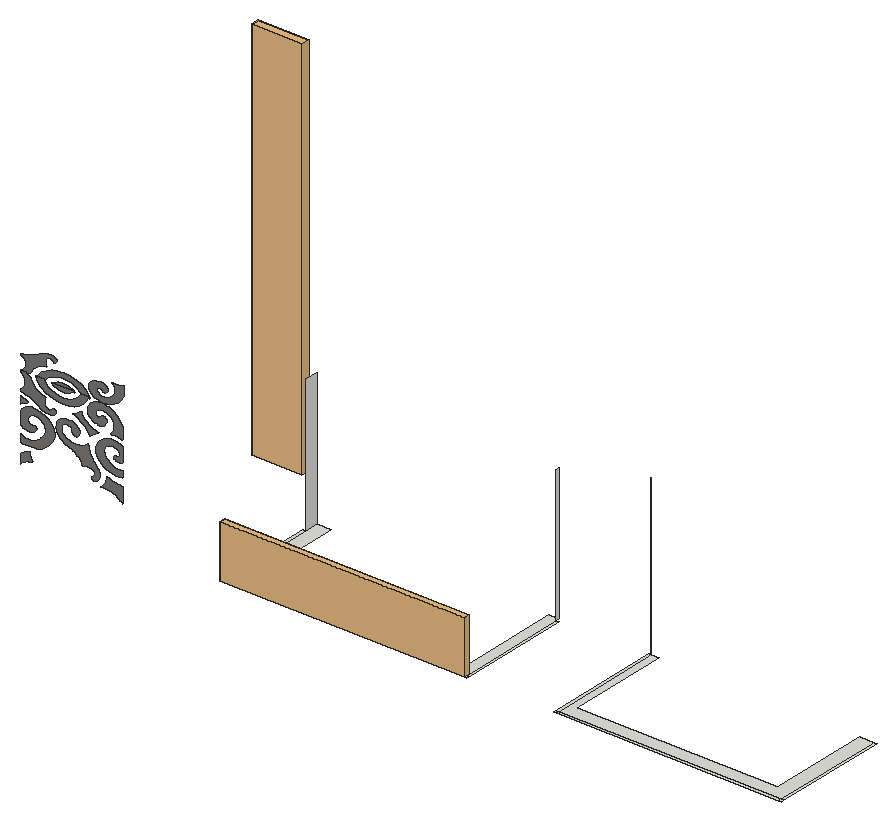
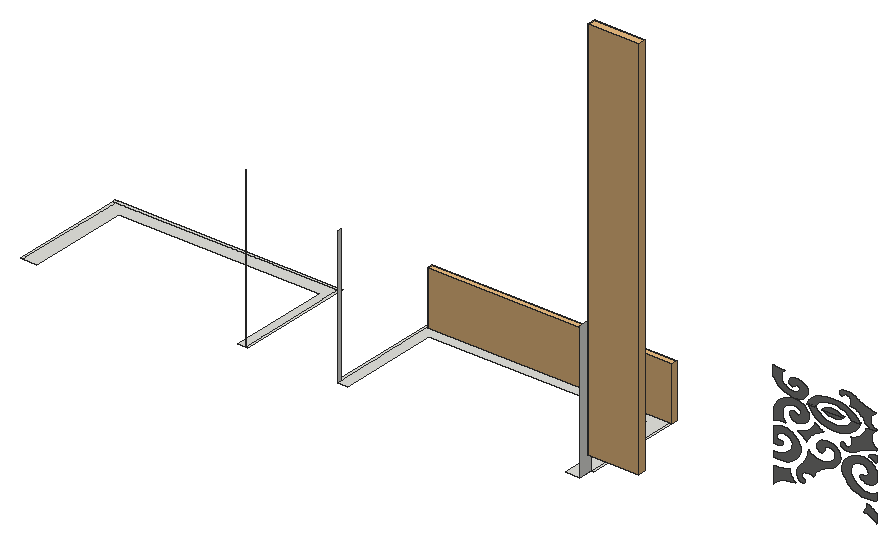
# SketchUp Ruby script. Lengths in inches.
U = 1.inch
M = Sketchup.active_model
def pt(a) = Geom::Point3d.new(a.map { |v| v * U })
def face(e, loops, mat)
  f = e.add_face(loops[0].map { |a| pt(a) })
  loops[1..].each { |l| e.add_face(l.map { |a| pt(a) }).erase! }
  f.material = f.back_material = mat if mat
  f
end
# faces: each face lists its corners as indices into pts; further lists are holes
def faces(e, pts, list, mat = nil) = list.each { |f| face(e, (f[0].is_a?(Array) ? f : [f]).map { |l| l.map { |i| pts[i] } }, mat) }
# xy, xz, yz: faces in a plane at the given z, y or x. An outline is a flat list of corners, or four numbers for a rectangle; further outlines are holes
def ring(l) = l.size == 4 ? [[l[0], l[1]], [l[2], l[1]], [l[2], l[3]], [l[0], l[3]]] : l.each_slice(2).to_a
def flat(e, list, mat, &to3) = list.each { |f| face(e, (f[0].is_a?(Array) ? f : [f]).map { |l| ring(l).map { |u, v| to3.(u, v) } }, mat) }
def xy(e, z, list, mat = nil) = flat(e, list, mat) { |x, y| [x, y, z] }
def xz(e, y, list, mat = nil) = flat(e, list, mat) { |x, z| [x, y, z] }
def yz(e, x, list, mat = nil) = flat(e, list, mat) { |y, z| [x, y, z] }
def lines(e, pts, list) = list.each { |a, b| e.add_line(pt(pts[a]), pt(pts[b])) }
# prism: a flat outline (further loops are holes) pulled along v
def prism(e, loops, v, mat = nil)
  f = face(e, loops, mat); d = Geom::Vector3d.new(v.map { |x| x * U })
  f.pushpull(f.normal.samedirection?(d) ? d.length : -d.length)
end
def box(e, o, s, mat = nil) = prism(e, [[o, [o[0] + s[0], o[1], o[2]], [o[0] + s[0], o[1] + s[1], o[2]], [o[0], o[1] + s[1], o[2]]]], [0, 0, s[2]], mat)
def at(x, y, z, deg = 0) = Geom::Transformation.translation(pt([x, y, z])) * Geom::Transformation.rotation(ORIGIN, Z_AXIS, deg.degrees)
def axes(o, x, y, z) = Geom::Transformation.new([*x, 0, *y, 0, *z, 0, *pt(o).to_a, 1])
def part(name) = M.definitions.add(name)
# library, detail: a bought-in or finely detailed component or shape, given as its bounding box
def library(name, o, s) = part(name).tap { |d| box(d.entities, o, s) }
def detail(e, o, s) = box(e.add_group.entities, o, s)
def put(e, d, t, mat = nil) = e.add_instance(d, t).tap { |i| i.material = mat if mat }
def group(e, t, mat = nil) = e.add_group.tap { |g| g.transformation = t; g.material = mat if mat }.entities
root = M.entities
M.materials.add("[0043_SaddleBrown]4").color = [124, 123, 122]
M.materials.add("[Granite Light Gray]").color = [149, 148, 144]
c1 = library("Scandinavian Door w/ Glass Wall\#2",[-41.94,78.85,0],[6.47,62.99,82.68])
c2 = library("Glass Railing",[0,0,0],[139.5,4.76,42])
xy(root,413.5,[[1800.63,557.9375,1993.07,559.875],[1993.07,557.9375,1995.01,559.875],[2063.58,557.9375,2065.52,559.875],[2065.52,557.9375,2240.81,559.875],[2240.81,557.9375,2242.75,559.875],
  [1800.45,559.875,1802.38,640.11],[1802.38,559.875,1993.07,559.875,1993.07,651.03,1985.21,651.03,1985.21,570.83,1813.71,570.83,1813.71,651.03,1802.38,651.03],[1993.07,559.875,1995.01,647.91],[2063.58,559.875,2065.52,651.03],[2065.52,559.875,2240.81,559.875,2240.81,651.03,2229.49,651.03,2229.49,570.83,2071.59,570.83,2071.59,651.03,2065.52,651.03],
  [2240.81,559.875,2242.75,651.03]])
xz(root,589.17,[[1698.99,418.4,1698.99,430.94,1697.95,430.96,1696.92,431.01,1695.88,431.09,1694.85,431.2,1693.83,431.34,1692.82,431.51,1691.82,431.7,1690.83,431.93,1689.85,432.18,1688.89,432.46,1687.9375,432.77,1687.01,433.11,1686.91,432.33,1686.75,431.56,1686.53,430.79,1686.27,430.03,1685.95,429.29,1685.57,428.55,1685.15,427.83,1684.68,427.13,1684.15,426.44,1683.58,425.78,1682.97,425.14,1682.31,424.52,1683.96,424.625,1685.62,424.61,1687.27,424.48,1688.89,424.22,1690.47,423.85,1691.99,423.36,1693.43,422.76,1694.78,422.0625,1696.02,421.27,1697.14,420.39,1698.14,419.43],[1618.6,418.5,1619.12,419.14,1619.71,419.74,1620.37,420.3125,1621.09,420.84,1621.86,421.32,1622.69,421.76,1623.57,422.14,1624.48,422.48,1625.43,422.75,1626.41,422.98,1627.41,423.14,1628.43,423.24,1628.01,423.73,1627.625,424.24,1627.28,424.76,1626.97,425.29,1626.7,425.83,1626.47,426.38,1626.28,426.94,1626.13,427.51,1626.02,428.08,1625.96,428.65,1625.93,429.23,1625.94,429.8,1625.25,429.54,1624.56,429.27,1623.89,428.97,1623.23,428.66,1622.59,428.33,1621.97,427.99,1621.36,427.63,1620.77,427.26,1620.2,426.87,1619.64,426.47,1619.11,426.05,1618.6,425.62],[1676.68,427.2,1677.23,427.23,1677.78,427.32,1678.3,427.46,1678.79,427.66,1679.23,427.9,1679.625,428.18,1679.96,428.51,1680.22,428.86,1680.41,429.24,1680.53,429.63,1680.57,430.04,1680.78,430.71,1680.93,431.38,1681,432.07,1681.01,432.76,1680.95,433.44,1680.82,434.125,1680.62,434.8,1680.35,435.46,1680.02,436.1,1679.62,436.72,1679.16,437.33,1678.64,437.9,1677.71,438.91,1676.84,439.95,1676.03,441.02,1675.29,442.11,1674.63,443.22,1674.03,444.36,1673.51,445.51,1673.05,446.68,1672.68,447.86,1672.375,449.05,1672.15,450.26,1672,451.46,1671.03,450.57,1669.91,449.77,1668.65,449.08,1667.29,448.52,1665.83,448.09,1664.31,447.8,1662.74,447.66,1661.17,447.66,1659.61,447.8125,1658.09,448.11,1656.63,448.54,1655.27,449.11,1654.29,449.65,1653.43,450.27,1652.68,450.97,1652.06,451.74,1651.58,452.55,1651.25,453.4,1651.07,454.28,1651.06,455.16,1651.2,456.04,1651.5,456.9,1651.94,457.72,1652.53,458.5,1653.08,458.79,1653.68,459.03,1654.32,459.19,1654.99,459.29,1655.68,459.31,1656.36,459.26,1657.02,459.13,1657.64,458.94,1658.23,458.68,1658.75,458.36,1659.19,457.99,1659.5625,457.57,1659.44,457.28,1659.35,456.98,1659.3,456.67,1659.28,456.37,1659.3,456.06,1659.34,455.75,1659.42,455.45,1659.54,455.16,1659.69,454.87,1659.86,454.59,1660.07,454.32,1660.31,454.0625,1660.54,453.87,1660.8125,453.7,1661.12,453.5625,1661.45,453.47,1661.8,453.41,1662.15,453.38,1662.51,453.41,1662.86,453.47,1663.19,453.5625,1663.5,453.7,1663.77,453.87,1664,454.0625,1664.67,454.87,1665.15,455.75,1665.4,456.67,1665.4375,457.61,1665.25,458.54,1664.84,459.4375,1664.23,460.27,1663.43,461.01,1662.46,461.64,1661.36,462.15,1660.16,462.51,1658.89,462.72,1657.47,462.91,1656.02,462.94,1654.59,462.8125,1653.2,462.53,1651.89,462.1,1650.68,461.53,1649.61,460.83,1648.69,460.03,1647.96,459.13,1647.42,458.17,1647.09,457.15,1646.98,456.12,1646.87,454.92,1646.93,453.72,1647.17,452.53,1647.57,451.37,1648.14,450.24,1648.86,449.16,1649.74,448.14,1650.76,447.19,1651.91,446.32,1653.18,445.55,1654.56,444.87,1656.02,444.3,1657.41,443.78,1658.74,443.1875,1660.02,442.53,1661.22,441.81,1662.35,441.03,1663.4,440.19,1664.37,439.31,1665.25,438.37,1666.03,437.39,1666.71,436.38,1667.3,435.33,1667.77,434.26,1668.45,434.625,1669.19,434.93,1669.98,435.15,1670.81,435.3,1671.65,435.36,1672.5,435.34,1673.34,435.24,1674.15,435.05,1674.92,434.79,1675.63,434.46,1676.28,434.06,1676.84,433.6,1677.05,433.23,1677.19,432.84,1677.28,432.45,1677.3,432.05,1677.26,431.65,1677.16,431.26,1677,430.875,1676.78,430.51,1676.5,430.16,1676.17,429.84,1675.79,429.55,1675.37,429.29,1675.14,429.13,1674.96,428.95,1674.83,428.75,1674.75,428.53,1674.74,428.3,1674.79,428.08,1674.9,427.87,1675.07,427.67,1675.28,427.51,1675.53,427.375,1675.82,427.28,1676.12,427.23],[1625.22,433.3,1627.48,433.36,1629.71,433.62,1631.89,434.07,1633.97,434.7,1635.9375,435.5,1637.76,436.47,1639.4,437.59,1640.85,438.85,1642.07,440.22,1643.74,442.26,1644.9,444.47,1645.51,446.8,1645.56,449.17,1645.03,451.51,1643.96,453.75,1642.37,455.82,1640.3125,457.67,1637.84,459.23,1635.03,460.46,1631.97,461.32,1628.75,461.79,1627.59,461.63,1626.46,461.4,1625.36,461.08,1624.3125,460.69,1623.32,460.24,1622.39,459.71,1621.53,459.125,1620.76,458.48,1620.07,457.79,1619.48,457.06,1618.99,456.28,1618.6,455.48,1618.6,447.4,1619.13,446.49,1619.91,445.68,1620.89,445,1622.05,444.48,1623.33,444.15,1624.68,444,1626.04,444.0625,1627.36,444.32,1628.57,444.76,1629.64,445.37,1630.51,446.13,1631.15,447,1631.24,447.21,1631.29,447.42,1631.3,447.64,1631.26,447.86,1631.17,448.07,1631.05,448.27,1630.88,448.46,1630.68,448.62,1630.45,448.76,1630.19,448.88,1629.91,448.97,1629.62,449.02,1628.89,448.93,1628.15,448.94,1627.43,449.05,1626.75,449.25,1626.13,449.54,1625.59,449.9,1625.16,450.33,1624.84,450.81,1624.65,451.32,1624.6,451.85,1624.68,452.38,1624.9,452.89,1625.08,453.55,1625.4,454.18,1625.86,454.77,1626.44,455.29,1627.13,455.75,1627.91,456.12,1628.76,456.4,1629.66,456.57,1630.59,456.65,1631.52,456.62,1632.43,456.48,1633.3,456.24,1634.66,455.45,1635.85,454.53,1636.84,453.51,1637.63,452.39,1638.1875,451.2,1638.5,449.96,1638.58,448.71,1638.4,447.46,1637.99,446.24,1637.33,445.08,1636.46,443.99,1635.38,443.01,1634.94,442.35,1634.43,441.73,1633.85,441.14,1633.2,440.59,1632.49,440.07,1631.72,439.6,1630.9,439.18,1630.04,438.8125,1629.14,438.49,1628.2,438.23,1627.23,438.03,1626.25,437.88,1625.55,437.82,1624.84,437.8,1624.14,437.83,1623.4375,437.89,1622.75,438,1622.07,438.16,1621.42,438.35,1620.79,438.58,1620.1875,438.85,1619.62,439.15,1619.09,439.48,1618.6,439.85,1618.6,434.28,1620.75,433.76,1622.96,433.44],[1696.39,436.71,1698.99,436.96,1698.99,441.66,1696.76,441.61,1694.55,441.84,1692.43,442.34,1690.46,443.09,1688.71,444.09,1687.22,445.28,1686.04,446.65,1685.21,448.14,1684.75,449.72,1684.67,451.32,1684.99,452.92,1685.6875,454.45,1686.48,455.1,1687.43,455.63,1688.51,456.03,1689.67,456.27,1690.87,456.35,1692.07,456.27,1693.23,456.02,1694.3,455.625,1695.25,455.09,1696.04,454.43,1696.65,453.68,1697.05,452.86,1697.125,452.53,1697.12,452.1875,1697.03,451.86,1696.87,451.54,1696.63,451.25,1696.33,450.99,1695.97,450.77,1695.5625,450.61,1695.125,450.49,1694.66,450.43,1694.2,450.42,1693.73,450.48,1693.49,450.4,1693.26,450.31,1693.05,450.19,1692.86,450.06,1692.68,449.92,1692.53,449.77,1692.4,449.6,1692.3,449.42,1692.22,449.24,1692.17,449.06,1692.15,448.87,1692.16,448.68,1692.53,448.29,1692.97,447.9375,1693.46,447.63,1694.01,447.38,1694.6,447.18,1695.23,447.04,1695.87,446.96,1696.52,446.9375,1697.17,446.98,1697.8,447.09,1698.42,447.25,1698.99,447.47,1698.99,459.11,1697.93,459.72,1696.77,460.23,1695.54,460.64,1694.24,460.9375,1692.91,461.12,1691.55,461.18,1690.19,461.12,1688.86,460.9375,1687.5625,460.64,1686.33,460.23,1685.17,459.72,1684.11,459.11,1683.22,458.48,1682.38,457.82,1681.61,457.11,1680.91,456.375,1680.28,455.6,1679.72,454.8,1679.23,453.97,1678.83,453.125,1678.5,452.26,1678.26,451.38,1678.09,450.49,1678.01,449.6,1678.13,447.71,1678.64,445.86,1679.53,444.08,1680.78,442.42,1682.36,440.92,1684.24,439.6,1686.37,438.5,1688.7,437.65,1691.19,437.06,1693.78,436.74],
  [1673.1,457.23,1673.65,457.6875,1674.21,458.14,1674.78,458.59,1675.36,459.03,1675.95,459.46,1676.55,459.89,1677.17,460.31,1677.79,460.72,1678.41,461.12,1679.05,461.52,1679.7,461.91,1680.36,462.29,1678.69,462.61,1677.08,463.04,1675.54,463.58,1674.08,464.23,1672.71,464.99,1671.46,465.83,1670.32,466.76,1669.32,467.77,1668.46,468.84,1667.74,469.96,1667.19,471.14,1666.8,472.34,1666.31,471.93,1665.8125,471.54,1665.29,471.16,1664.75,470.79,1664.1875,470.43,1663.61,470.09,1663.01,469.77,1662.4,469.47,1661.77,469.18,1661.13,468.9,1660.48,468.65,1659.8125,468.41,1661.375,467.83,1662.88,467.18,1664.3125,466.45,1665.67,465.65,1666.95,464.79,1668.14,463.86,1669.23,462.87,1670.22,461.83,1671.11,460.74,1671.89,459.6,1672.55,458.43],[1618.6,460.92,1619.02,461.25,1619.45,461.57,1619.91,461.88,1620.38,462.17,1620.875,462.45,1621.38,462.71,1621.9,462.95,1622.44,463.18,1622.99,463.39,1623.56,463.58,1624.13,463.75,1624.72,463.91,1624.34,464.24,1623.92,464.55,1623.48,464.84,1623.02,465.11,1622.52,465.35,1622.01,465.56,1621.47,465.76,1620.92,465.92,1620.36,466.05,1619.78,466.16,1619.19,466.24,1618.6,466.28],[1640.65,461.65,1641.57,461.6875,1642.48,461.8,1643.37,461.98,1644.23,462.23,1644.53,462.34,1644.82,462.47,1645.1,462.62,1645.35,462.79,1645.59,462.96,1645.8,463.16,1645.99,463.36,1646.16,463.58,1646.3,463.8,1646.42,464.03,1646.51,464.27,1646.57,464.52,1646.59,464.75,1646.58,464.99,1646.53,465.23,1646.44,465.46,1646.32,465.6875,1646.16,465.9,1645.97,466.1,1645.75,466.28,1645.5,466.4375,1645.23,466.58,1644.9375,466.69,1644.63,466.78,1644.4375,466.54,1644.23,466.29,1644.02,466.06,1643.79,465.83,1643.55,465.6,1643.3,465.38,1643.04,465.17,1642.77,464.96,1642.49,464.77,1642.2,464.57,1641.91,464.39,1641.6,464.21,1641.17,464.28,1640.76,464.375,1640.36,464.5,1639.98,464.65,1639.625,464.83,1639.29,465.03,1638.99,465.26,1638.72,465.5,1638.48,465.77,1638.28,466.04,1638.12,466.33,1637.99,466.63,1637.85,467.11,1637.74,467.58,1637.67,468.0625,1637.62,468.55,1637.61,469.03,1637.63,469.51,1637.6875,469.99,1637.77,470.47,1637.89,470.95,1638.04,471.42,1638.23,471.88,1638.44,472.34,1636.97,472.75,1635.5625,473.24,1634.21,473.83,1632.95,474.5,1631.76,475.24,1630.68,476.0625,1629.7,476.95,1628.84,477.9,1628.09,478.89,1627.47,479.94,1626.99,481.01,1626.63,482.12,1626.25,482.3,1625.88,482.48,1625.16,482.88,1624.8125,483.09,1624.47,483.31,1624.14,483.53,1623.82,483.77,1623.51,484.01,1623.22,484.25,1622.93,484.5,1622.65,484.8,1618.6,484.8,1618.6,483.92,1619.6875,483.03,1620.6,482.05,1621.33,480.99,1621.86,479.87,1622.1875,478.71,1622.29,477.53,1622.1875,476.35,1621.86,475.1875,1621.33,474.07,1620.6,473.01,1619.6875,472.02,1618.6,471.14,1618.6,469.95,1620.07,469.73,1621.53,469.45,1622.96,469.11,1624.36,468.72,1625.73,468.27,1627.07,467.77,1628.36,467.21,1629.61,466.61,1630.8125,465.96,1631.96,465.26,1633.06,464.51,1634.09,463.73,1634.75,463.26,1635.46,462.84,1636.24,462.48,1637.0625,462.18,1637.93,461.94,1638.82,461.77,1639.73,461.68],[1698.99,463.51,1698.99,472.52,1698.58,473.85,1697.98,475.15,1697.22,476.4,1696.3,477.6,1695.21,478.72,1693.99,479.76,1692.63,480.71,1691.15,481.57,1689.56,482.3125,1687.88,482.95,1686.125,483.46,1684.31,483.85,1682.64,483.91,1680.98,483.79,1679.36,483.49,1677.82,483.03,1676.4,482.4,1675.11,481.63,1674.01,480.73,1673.09,479.72,1672.4,478.625,1671.94,477.47,1671.72,476.28,1671.75,475.07,1671.7,474.3125,1671.79,473.55,1671.99,472.81,1672.33,472.09,1672.78,471.4,1673.34,470.76,1674.01,470.17,1674.78,469.64,1675.62,469.1875,1676.54,468.81,1677.51,468.51,1678.53,468.31,1679.2,468.02,1679.94,467.82,1680.71,467.71,1681.5,467.7,1682.28,467.78,1683.02,467.96,1683.72,468.22,1684.34,468.57,1684.87,468.99,1685.29,469.47,1685.6,469.99,1685.77,470.54,1686.17,470.95,1686.47,471.4,1686.65,471.88,1686.72,472.38,1686.66,472.88,1686.49,473.36,1686.21,473.81,1685.82,474.23,1685.34,474.59,1684.78,474.88,1684.16,475.1,1683.5,475.24,1683.26,474.99,1683.02,474.75,1682.5,474.29,1682.22,474.07,1681.9375,473.85,1681.64,473.64,1681.34,473.44,1681.02,473.25,1680.7,473.0625,1680.37,472.88,1680.03,472.71,1679.66,472.88,1679.31,473.08,1679,473.31,1678.72,473.55,1678.48,473.82,1678.28,474.1,1678.13,474.4,1678.02,474.71,1677.96,475.02,1677.94,475.34,1677.97,475.66,1678.06,475.97,1678.34,476.6,1678.77,477.18,1679.3125,477.71,1679.97,478.17,1680.73,478.54,1681.55,478.83,1682.43,479.01,1683.34,479.09,1684.26,479.06,1685.16,478.93,1686.01,478.7,1686.8,478.36,1688.22,477.55,1689.47,476.6,1690.53,475.54,1691.39,474.39,1692.01,473.16,1692.41,471.88,1692.56,470.58,1692.46,469.28,1692.125,467.99,1691.55,466.75,1690.75,465.58,1689.73,464.5,1690.51,464.63,1691.3,464.73,1692.1,464.78,1692.91,464.8,1693.71,464.77,1694.51,464.71,1695.3,464.6,1696.07,464.46,1696.83,464.28,1697.58,464.06,1698.3,463.8],[1651.83,472.34,1656.66,472.75,1661.22,473.95,1665.27,475.88,1668.6,478.43,1671.04,481.46,1672.4375,484.8,1666.28,484.8,1665.1,482.62,1663.29,480.66,1660.94,479.03,1658.16,477.8,1655.07,477.04,1651.83,476.77,1648.58,477.02,1645.49,477.76,1642.6875,478.97,1640.32,480.59,1638.48,482.53,1637.28,484.8,1631.12,484.8,1632.55,481.37,1635.01,478.35,1638.36,475.82,1642.4375,473.91,1647.01,472.73],
  [1652.15,480.9,1653.91,481.02,1655.61,481.375,1657.1875,481.95,1658.58,482.74,1659.75,483.7,1660.65,484.8,1643.65,484.8,1644.55,483.7,1645.71,482.74,1647.11,481.95,1648.6875,481.375,1650.39,481.02],[1619.31,483.9,1619.31,484.65,1620.39,485.41,1621.3125,486.24,1622.04,487.15,1622.57,488.1,1622.89,489.09,1623,490.1,1622.89,491.1,1622.57,492.09,1622.04,493.05,1621.3125,493.95,1620.39,494.79,1619.31,495.54,1619.31,496.56,1620.78,496.75,1622.23,496.98,1623.67,497.27,1625.07,497.61,1626.4375,497.99,1627.77,498.41,1629.07,498.89,1630.32,499.4,1631.52,499.96,1632.67,500.55,1633.76,501.1875,1634.8,501.86,1635.45,502.26,1636.17,502.61,1636.95,502.92,1637.77,503.18,1638.63,503.375,1639.53,503.52,1640.4375,503.6,1641.36,503.63,1642.28,503.59,1643.19,503.5,1644.08,503.34,1644.93,503.13,1645.24,503.04,1645.53,502.92,1645.8,502.8,1646.06,502.66,1646.29,502.51,1646.51,502.34,1646.7,502.17,1646.87,501.98,1647.01,501.79,1647.125,501.59,1647.21,501.39,1647.27,501.18,1647.3,500.98,1647.29,500.78,1647.24,500.57,1647.15,500.375,1647.03,500.1875,1646.87,500.01,1646.68,499.84,1646.46,499.68,1646.21,499.55,1645.9375,499.43,1645.65,499.33,1645.34,499.25,1644.94,499.67,1644.5,500.07,1644.26,500.26,1644.01,500.44,1643.75,500.625,1643.48,500.8,1643.2,500.97,1642.91,501.13,1642.61,501.29,1642.31,501.44,1641.88,501.38,1641.47,501.3,1641.07,501.2,1640.69,501.07,1640.33,500.91,1640,500.74,1639.7,500.55,1639.43,500.34,1639.1875,500.12,1638.99,499.88,1638.82,499.64,1638.7,499.38,1638.56,498.98,1638.45,498.57,1638.375,498.16,1638.33,497.75,1638.32,497.34,1638.34,496.93,1638.39,496.52,1638.48,496.11,1638.6,495.7,1638.75,495.3,1638.93,494.91,1639.15,494.52,1637.68,494.17,1636.27,493.75,1634.92,493.25,1633.65,492.68,1632.47,492.05,1631.39,491.35,1630.41,490.59,1629.54,489.78,1628.8,488.93,1628.18,488.05,1627.69,487.13,1627.34,486.1875,1626.96,486.04,1626.59,485.88,1626.22,485.71,1625.87,485.54,1625.52,485.36,1625.18,485.17,1624.85,484.98,1624.53,484.78,1624.22,484.58,1623.92,484.37,1623.63,484.16,1623.35,483.9],[1631.83,483.9,1633.26,486.82,1635.72,489.4,1639.07,491.55,1643.14,493.18,1647.71,494.1875,1652.54,494.52,1657.36,494.17,1661.92,493.14,1665.98,491.5,1669.3125,489.33,1671.74,486.75,1673.15,483.9,1666.99,483.9,1665.81,485.76,1664,487.43,1661.65,488.82,1658.86,489.86,1655.78,490.51,1652.54,490.74,1649.29,490.53,1646.2,489.9,1643.4,488.87,1641.02,487.49,1639.19,485.83,1637.98,483.9],[1644.36,483.9,1645.25,484.84,1646.42,485.66,1647.82,486.33,1649.39,486.82,1651.09,487.125,1652.86,487.23,1654.62,487.125,1656.32,486.82,1657.9,486.33,1659.29,485.66,1660.46,484.84,1661.35,483.9],[1683.35,484.66,1681.6875,484.76,1680.07,485.02,1678.53,485.41,1677.1,485.95,1675.82,486.6,1674.71,487.37,1673.8,488.23,1673.11,489.16,1672.65,490.15,1672.43,491.16,1672.46,492.1875,1672.41,492.84,1672.49,493.48,1672.7,494.12,1673.03,494.73,1673.49,495.32,1674.05,495.87,1674.72,496.37,1675.48,496.82,1676.33,497.21,1677.25,497.53,1678.22,497.78,1679.24,497.95,1679.91,498.2,1680.65,498.37,1681.42,498.46,1682.21,498.48,1682.98,498.4,1683.73,498.25,1684.42,498.02,1685.05,497.73,1685.58,497.37,1686,496.96,1686.3,496.52,1686.48,496.05,1686.88,495.7,1687.18,495.32,1687.36,494.91,1687.43,494.48,1687.37,494.0625,1687.2,493.65,1686.92,493.26,1686.53,492.91,1686.05,492.6,1685.49,492.35,1684.87,492.17,1684.2,492.05,1683.97,492.26,1683.73,492.46,1683.21,492.86,1682.93,493.05,1682.35,493.41,1682.04,493.58,1681.73,493.74,1681.41,493.9,1681.07,494.05,1680.74,494.2,1680.36,494.05,1680.02,493.89,1679.7,493.7,1679.43,493.49,1679.1875,493.26,1678.99,493.02,1678.83,492.76,1678.73,492.5,1678.66,492.23,1678.65,491.96,1678.68,491.69,1678.76,491.43,1679.05,490.89,1679.47,490.39,1680.02,489.94,1680.68,489.55,1681.43,489.23,1682.26,488.99,1683.14,488.83,1684.05,488.77,1684.97,488.79,1685.86,488.9,1686.72,489.1,1687.51,489.39,1688.93,490.08,1690.18,490.89,1691.24,491.79,1692.09,492.77,1692.72,493.82,1693.12,494.91,1693.27,496.02,1693.17,497.13,1692.83,498.22,1692.26,499.28,1691.45,500.28,1690.44,501.2,1691.22,501.09,1692.01,501.01,1692.8125,500.96,1693.61,500.95,1694.42,500.97,1695.21,501.02,1696,501.11,1696.78,501.23,1697.54,501.39,1698.28,501.57,1699,501.79,1699.7,502.04,1699.7,494.37,1699.28,493.23,1698.69,492.125,1697.93,491.06,1697,490.04,1695.92,489.08,1694.7,488.2,1693.34,487.38,1691.86,486.66,1690.27,486.02,1688.59,485.48,1686.83,485.04,1685.01,484.71]],"[0043_SaddleBrown]4")
xz(root,651.03,[[2065.31,413.5,2065.52,538.1875]])
yz(root,1802.38,[[640.11,413.5,651.03,520.4375]])
yz(root,1993.07,[[647.91,413.5,651.03,520.4375]])
p = [[1618.6,589.17,469.95],[1618.6,589.17,466.28]]
lines(root,p,[[0,1]])
put(root,c1,axes([1696.87,621.1,440.32],[0,-1,0],[0.63229,0,0],[0,0,3.672]))
put(root,c2,axes([1800.63,557.9375,413.5],[1.37946,0,0],[0,1,0],[0,0,1]),"[Granite Light Gray]")
